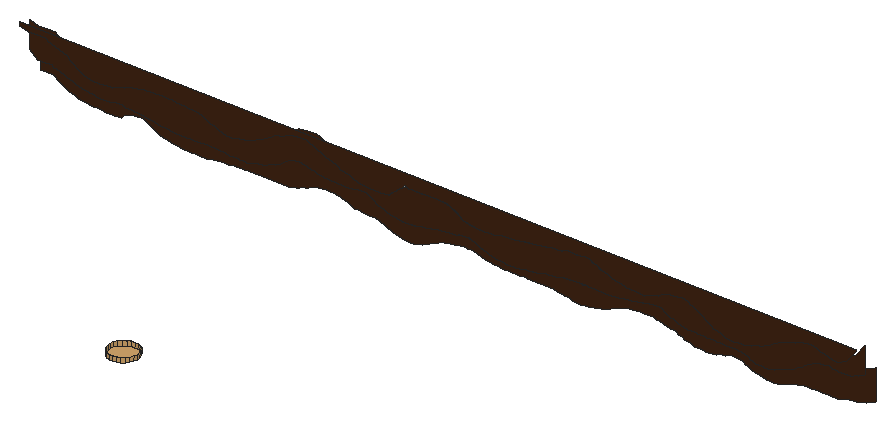
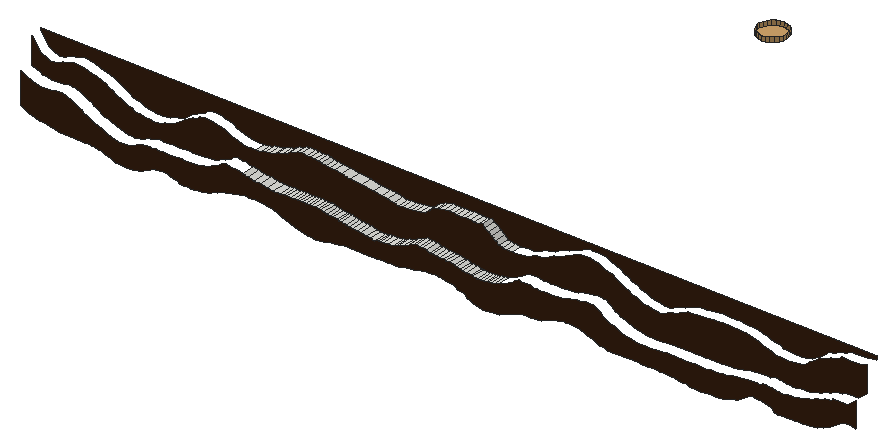
# SketchUp Ruby script. Lengths in inches.
U = 1.inch
M = Sketchup.active_model
def pt(a) = Geom::Point3d.new(a.map { |v| v * U })
def face(e, loops, mat)
  f = e.add_face(loops[0].map { |a| pt(a) })
  loops[1..].each { |l| e.add_face(l.map { |a| pt(a) }).erase! }
  f.material = f.back_material = mat if mat
  f
end
# faces: each face lists its corners as indices into pts; further lists are holes
def faces(e, pts, list, mat = nil) = list.each { |f| face(e, (f[0].is_a?(Array) ? f : [f]).map { |l| l.map { |i| pts[i] } }, mat) }
# xy, xz, yz: faces in a plane at the given z, y or x. An outline is a flat list of corners, or four numbers for a rectangle; further outlines are holes
def ring(l) = l.size == 4 ? [[l[0], l[1]], [l[2], l[1]], [l[2], l[3]], [l[0], l[3]]] : l.each_slice(2).to_a
def flat(e, list, mat, &to3) = list.each { |f| face(e, (f[0].is_a?(Array) ? f : [f]).map { |l| ring(l).map { |u, v| to3.(u, v) } }, mat) }
def xy(e, z, list, mat = nil) = flat(e, list, mat) { |x, y| [x, y, z] }
def xz(e, y, list, mat = nil) = flat(e, list, mat) { |x, z| [x, y, z] }
def yz(e, x, list, mat = nil) = flat(e, list, mat) { |y, z| [x, y, z] }
def lines(e, pts, list) = list.each { |a, b| e.add_line(pt(pts[a]), pt(pts[b])) }
# prism: a flat outline (further loops are holes) pulled along v
def prism(e, loops, v, mat = nil)
  f = face(e, loops, mat); d = Geom::Vector3d.new(v.map { |x| x * U })
  f.pushpull(f.normal.samedirection?(d) ? d.length : -d.length)
end
def box(e, o, s, mat = nil) = prism(e, [[o, [o[0] + s[0], o[1], o[2]], [o[0] + s[0], o[1] + s[1], o[2]], [o[0], o[1] + s[1], o[2]]]], [0, 0, s[2]], mat)
def at(x, y, z, deg = 0) = Geom::Transformation.translation(pt([x, y, z])) * Geom::Transformation.rotation(ORIGIN, Z_AXIS, deg.degrees)
def axes(o, x, y, z) = Geom::Transformation.new([*x, 0, *y, 0, *z, 0, *pt(o).to_a, 1])
def part(name) = M.definitions.add(name)
# library, detail: a bought-in or finely detailed component or shape, given as its bounding box
def library(name, o, s) = part(name).tap { |d| box(d.entities, o, s) }
def detail(e, o, s) = box(e.add_group.entities, o, s)
def put(e, d, t, mat = nil) = e.add_instance(d, t).tap { |i| i.material = mat if mat }
def group(e, t, mat = nil) = e.add_group.tap { |g| g.transformation = t; g.material = mat if mat }.entities
root = M.entities
M.materials.add("[Field Square Tile]").color = [211, 167, 108]
M.materials.add("[Wood Veneer 01]").color = [66, 38, 20]
xy(root,243.05,[[2994.54,563.18,2995.22,565.74]])
xy(root,243.07,[[2992.6875,563.18,2993.27,565.74]])
xy(root,243.09,[[2989.375,563.18,2989.9,565.74],[2989.9,563.18,2990.42,565.74],[2990.42,563.18,2991.08,565.74],[2991.08,563.18,2991.53,565.74]])
xy(root,249.21,[[2962.17,561.05,2963.06,563.18]])
xy(root,249.22,[[2963.78,561.05,2964.6875,563.18]])
xy(root,249.23,[[2965.33,561.05,2966.23,563.18]])
xy(root,250.6875,[[2960.72,492.77,2960.06,492.86,2959.44,493.11,2958.91,493.52,2958.5,494.05,2958.25,494.67,2958.16,495.33,2958.25,495.99,2958.5,496.61,2958.91,497.14,2959.44,497.55,2960.06,497.81,2960.72,497.89,2961.38,497.81,2962,497.55,2962.53,497.14,2962.94,496.61,2963.2,495.99,2963.28,495.33,2963.2,494.67,2962.94,494.05,2962.53,493.52,2962,493.11,2961.38,492.86]],"[Field Square Tile]")
xz(root,561.05,[[3020.59,244.87,3021.5,245.01,3022.4375,245.12,3023.2,245.25,3023.96,245.41,3024.59,245.78,3025.39,245.88,3026.1,246.16,3026.7,246.57,3027.49,246.9,3028.09,247.35,3028.76,247.62,3029.35,248.06,3030.11,248.32,3031.22,248.66,3032,248.79,3032.86,249.19,3033.53,249.32,3034.46,249.41,3035.31,249.48,3036.06,249.21,3036.7,248.96,3037.4,248.9,3038.2,248.42,3038.91,248.3,3039.62,248.22,3040.4375,248.56,3041.37,249.02,3043.1,251.16,3043.1,251.5,2889.09,251.5,2889.09,250.88,2890.68,250.53,2892.3,250.54,2893.76,250.55,2894.29,250.15,2894.9,249.97,2895.7,249.8,2896.37,249.41,2897.04,249.2,2897.81,249.01,2898.3,248.51,2898.93,248.07,2899.58,247.72,2900.22,247.25,2900.77,246.88,2901.49,246.73,2902.15,246.62,2902.89,246.54,2903.67,246.51,2904.45,246.58,2905.25,246.59,2906.05,246.69,2906.76,247.03,2907.45,247.2,2908.42,247.39,2909.05,247.78,2909.83,247.89,2910.83,248.18,2911.47,248.29,2912.36,248.35,2913.09,248.4,2914.08,248.4375,2914.74,248.46,2915.63,248.47,2916.37,248.48,2917.26,248.49,2917.99,248.39,2919.39,248.28,2920.42,248.15,2921.24,248.11,2922.04,248.08,2922.88,247.66,2923.51,247.46,2924.19,247.08,2924.875,246.94,2925.73,246.66,2926.34,246.35,2927.11,246.05,2928.01,246.13,2928.72,246.29,2929.52,246.41,2930.43,246.55,2931.16,246.92,2931.77,247.12,2932.45,247.31,2933.02,247.71,2933.95,248.03,2934.66,248.46,2935.44,248.82,2936.16,249.37,2936.95,249.5625,2937.85,249.9,2938.77,250.35,2939.43,250.49,2940.24,250.6,2941.26,250.58,2941.9,250.61,2942.52,250.32,2943.21,250.0625,2943.87,249.68,2944.63,249.46,2945.52,248.95,2946.74,248.69,2947.65,248.26,2948.25,247.9,2949.38,247.66,2949.96,247.53,2950.64,247.25,2951.45,246.95,2952.14,246.75,2952.93,246.66,2953.64,246.59,2954.53,246.55,2955.46,246.63,2956.2,246.74,2956.93,246.87,2957.54,247.42,2958.21,247.96,2958.78,248.44,2959.52,248.85,2959.99,249.34,2960.72,249.125,2961.49,249.17,2962.17,249.21,2963.06,249.21,2963.78,249.22,2964.6875,249.22,2965.33,249.23,2966.23,249.23,2966.97,249.24,2967.77,249.14,2968.4,248.82,2969.19,248.54,2969.89,248.04,2970.58,247.48,2971.47,247.29,2972.29,247.15,2973.02,247.05,2973.74,247,2974.65,246.96,2975.375,246.94,2976.29,247.04,2977.35,247.36,2978.53,247.43,2980.18,247.6,2982.16,247.98,2984.36,248.1875,2985.97,248.49,2987.22,248.62,2988.16,248.69,2988.84,248.75,2989.5,249.09,2990.2,249.18,2990.98,249.13,2991.68,249.17,2992.38,249.18,2993.28,249.29,2994.01,249.21,2994.62,248.8,2995.3125,248.73,2996.09,248.26,2996.79,248.02,2997.59,247.8125,2998.3,247.4,2999.21,247.27,2999.95,247.18,3000.875,246.91,3001.74,246.84,3002.69,246.79,3003.47,246.75,3004.22,246.83,3005.26,247.25,3006.13,247.55,3006.8,247.66,3007.43,248.16,3008.22,248.41,3008.92,248.52,3009.62,248.72,3010.32,248.8,3011.21,248.85,3012.04,248.6875,3012.58,248.26,3013.27,248.06,3014.16,247.55,3014.87,247.19,3015.68,246.63,3016.3125,246.13,3016.9,245.83,3017.58,245.67,3018.45,245.46,3019.16,245.0625,3019.875,244.95]],"[Wood Veneer 01]")
xz(root,563.18,[[3024.59,241.09,3025.16,241.14,3025.8,241.35,3026.39,241.46,3027.33,241.85,3028.33,242.23,3028.89,242.42,3029.61,242.61,3030.125,242.91,3030.5,243.14,3031.04,243.52,3031.52,243.71,3031.85,244.02,3032.29,244.21,3032.88,244.57,3033.35,244.76,3033.97,245.125,3034.47,245.32,3034.95,245.41,3035.5,245.48,3035.99,245.59,3036.52,245.55,3037.13,245.35,3037.62,245.31,3038.17,245.27,3038.73,245.24,3039.29,245.22,3039.85,245.34,3040.48,245.42,3041.0625,245.52,3041.44,245.76,3041.91,245.9,3043.1,246.43,3043.1,251.16,3041.37,249.02,3040.4375,248.56,3039.62,248.22,3038.91,248.3,3038.2,248.42,3037.4,248.9,3036.7,248.96,3036.06,249.21,3035.31,249.48,3034.46,249.41,3033.53,249.32,3032.86,249.19,3032,248.79,3031.22,248.66,3030.11,248.32,3029.35,248.06,3028.76,247.62,3028.09,247.35,3027.49,246.9,3026.7,246.57,3026.1,246.16,3025.39,245.88,3024.59,245.78,3023.96,245.41,3023.2,245.25,3022.4375,245.12,3021.5,245.01,3020.59,244.87,3019.875,244.95,3019.16,245.0625,3018.45,245.46,3017.58,245.67,3016.9,245.83,3016.3125,246.13,3015.68,246.63,3014.87,247.19,3014.16,247.55,3013.27,248.06,3012.58,248.26,3012.04,248.6875,3011.21,248.85,3010.32,248.8,3009.62,248.72,3008.92,248.52,3008.22,248.41,3007.43,248.16,3006.8,247.66,3006.13,247.55,3005.26,247.25,3004.22,246.83,3003.47,246.75,3002.69,246.79,3001.74,246.84,3000.875,246.91,2999.95,247.18,2999.21,247.27,2998.3,247.4,2997.59,247.8125,2996.79,248.02,2996.09,248.26,2995.3125,248.73,2994.62,248.8,2994.01,249.21,2993.28,249.29,2992.38,249.18,2991.68,249.17,2990.98,249.13,2990.2,249.18,2989.5,249.09,2988.84,248.75,2988.16,248.69,2987.22,248.62,2985.97,248.49,2984.36,248.1875,2982.16,247.98,2980.18,247.6,2978.53,247.43,2977.35,247.36,2976.29,247.04,2975.375,246.94,2974.65,246.96,2973.74,247,2973.02,247.05,2972.29,247.15,2971.47,247.29,2970.58,247.48,2969.89,248.04,2969.19,248.54,2968.4,248.82,2967.77,249.14,2966.97,249.24,2966.23,249.23,2965.33,249.23,2964.6875,249.22,2963.78,249.22,2963.06,249.21,2962.17,249.21,2961.49,249.17,2960.72,249.125,2959.99,249.34,2959.52,248.85,2958.78,248.44,2958.21,247.96,2957.54,247.42,2956.93,246.87,2956.2,246.74,2955.46,246.63,2954.53,246.55,2953.64,246.59,2952.93,246.66,2952.14,246.75,2951.45,246.95,2950.64,247.25,2949.96,247.53,2949.38,247.66,2948.25,247.9,2947.65,248.26,2946.74,248.69,2945.52,248.95,2944.63,249.46,2943.87,249.68,2943.21,250.0625,2942.52,250.32,2941.9,250.61,2941.26,250.58,2940.24,250.6,2939.43,250.49,2938.77,250.35,2937.85,249.9,2936.95,249.5625,2936.16,249.37,2935.44,248.82,2934.66,248.46,2933.95,248.03,2933.02,247.71,2932.45,247.31,2931.77,247.12,2931.16,246.92,2930.43,246.55,2929.52,246.41,2928.72,246.29,2928.01,246.13,2927.11,246.05,2926.34,246.35,2925.73,246.66,2924.875,246.94,2924.19,247.08,2923.51,247.46,2922.88,247.66,2922.04,248.08,2921.24,248.11,2920.42,248.15,2919.39,248.28,2917.99,248.39,2917.26,248.49,2916.37,248.48,2915.63,248.47,2914.74,248.46,2914.08,248.4375,2913.09,248.4,2912.36,248.35,2911.47,248.29,2910.83,248.18,2909.83,247.89,2909.05,247.78,2908.42,247.39,2907.45,247.2,2906.76,247.03,2906.05,246.69,2905.25,246.59,2904.45,246.58,2903.67,246.51,2902.89,246.54,2902.15,246.62,2901.49,246.73,2900.77,246.88,2900.22,247.25,2899.58,247.72,2898.93,248.07,2898.3,248.51,2897.81,249.01,2897.04,249.2,2896.37,249.41,2895.7,249.8,2894.9,249.97,2894.29,250.15,2893.76,250.55,2892.3,250.54,2890.68,250.53,2889.09,250.88,2889.09,246.2,2890.66,244.96,2892.05,244.9375,2893.3,244.92,2893.52,244.61,2894.08,244.54,2894.84,244.41,2895.51,244.11,2896.03,243.95,2896.69,243.79,2897.21,243.48,2897.85,243.3,2898.4375,243.14,2898.92,243.06,2899.64,242.85,2900.22,242.78,2901.03,242.73,2901.57,242.68,2902.24,242.51,2902.76,242.46,2903.3,242.58,2903.93,242.57,2904.56,242.81,2905.13,242.86,2905.69,242.89,2906.33,242.92,2906.76,242.625,2907.37,242.65,2907.92,242.62,2908.55,242.58,2909.11,242.57,2909.75,242.48,2910.41,242.38,2911.07,242.34,2911.74,242.24,2912.91,241.96,2913.68,241.89,2914.5,241.83,2915.1,241.78,2915.87,241.75,2916.32,241.74,2916.87,241.72,2918.13,241.7,2918.86,241.69,2919.53,241.68,2920.12,241.68,2920.61,241.67,2921.3125,241.74,2921.88,241.75,2923.88,241.75,2924.37,241.67,2924.9,241.66,2925.51,241.57,2926.05,241.53,2926.67,241.51,2927.22,241.49,2927.92,241.48,2928.58,241.47,2929.15,241.46,2929.86,241.6,2930.59,241.85,2931.26,241.91,2932.16,242.1,2932.93,242.46,2933.63,242.78,2934.4,242.97,2934.93,243.23,2935.33,243.48,2935.85,243.72,2936.1875,244.12,2936.66,244.39,2937.14,244.73,2937.625,244.87,2938.21,244.95,2938.89,245.01,2939.54,244.81,2940.11,244.7,2940.59,244.67,2941.2,244.55,2941.74,244.51,2942.2,244.25,2942.95,244.11,2943.51,244.04,2944.13,243.99,2944.85,243.95,2945.35,243.93,2946.04,243.91,2946.61,243.89,2947.31,243.88,2947.96,243.94,2948.6,243.95,2949.16,244.1,2949.79,244.13,2950.27,244.15,2950.79,244.17,2951.31,244.18,2951.91,243.8,2952.45,243.43,2953.06,243.09,2953.45,242.875,2953.95,242.68,2954.54,242.51,2955.05,242.21,2955.65,242.11,2956.33,241.96,2956.89,241.89,2957.35,241.85,2957.87,241.8125,2958.38,241.79,2958.96,241.78,2959.63,241.91,2960.1,241.93,2960.77,242.09,2961.54,242.2,2962.04,242.24,2962.65,242.42,2963.2,242.47,2963.95,242.71,2964.59,242.78,2965.07,242.82,2965.76,242.85,2966.46,242.87,2967.01,243.02,2967.63,243.05,2968.18,243.29,2968.86,243.35,2969.41,243.39,2970.01,243.42,2970.78,243.14,2971.35,242.9375,2971.9,242.65,2972.52,242.39,2973.28,242.14,2973.92,241.89,2974.41,241.78,2975.46,241.63,2976.23,241.56,2976.83,241.51,2977.28,241.48,2977.8,241.46,2978.67,241.51,2979.39,241.59,2980.33,241.82,2981.11,241.87,2981.875,241.98,2982.49,242.02,2983.14,242.19,2983.84,242.38,2984.33,242.4375,2984.85,242.48,2985.51,242.58,2986.04,242.61,2986.625,242.77,2987.08,242.95,2987.64,243.01,2988.15,243.05,2988.72,243.08,2989.375,243.09,2991.53,243.09,2992.1,243.08,2992.6875,243.07,2993.27,243.07,2993.93,243.0625,2994.54,243.05,2995.22,243.05,2996.49,243.1,2997.66,243.17,2998.8,243.4,3000.0625,243.52,3001.19,243.71,3002.09,243.99,3002.79,244.08,3003.49,244.21,3004.07,244.27,3004.61,244.3,3005.28,244.39,3005.875,244.19,3006.25,243.88,3006.73,243.59,3007.28,243.33,3007.83,243.22,3008.32,242.92,3008.8,242.75,3009.36,242.6,3009.92,242.52,3010.48,242.47,3011.0625,242.43,3011.64,242.4,3012.22,242.39,3012.8,242.37,3013.38,242.36,3013.97,242.35,3015.13,242.33,3015.71,242.33,3016.43,242.32,3016.9,242.3125,3017.54,242.3,3018.21,242.3,3018.66,242.29,3019.3,242.28,3019.8125,242.28,3020.44,242.2,3021.02,241.97,3021.59,241.84,3022.1,241.57,3022.52,241.33,3022.99,241.24,3023.52,241.17,3023.99,241.12]],"[Wood Veneer 01]")
xz(root,565.74,[[2957.95,236.98,2958.63,237.22,2959.48,237.43,2960.1,237.74,2960.8,238.02,2961.24,238.375,2961.8,238.51,2962.4375,238.76,2963.08,239.12,2963.66,239.22,2964.66,239.31,2965.47,239.54,2965.96,239.6,2966.58,239.65,2967.17,239.69,2967.73,239.7,2968.46,239.72,2969.07,239.56,2969.74,239.44,2970.59,239.16,2971.14,239.07,2971.91,238.93,2972.79,238.78,2973.27,238.73,2973.94,238.6875,2974.63,238.66,2975.3,238.65,2976.08,238.64,2976.7,238.63,2977.39,238.625,2978.25,238.625,2978.81,238.62,2983.7,238.62,2984.39,238.45,2985.15,238.25,2985.77,238.19,2986.54,238.15,2987.17,237.86,2987.94,237.79,2988.65,237.74,2989.52,237.87,2990.17,237.88,2991.29,238.14,2992.51,238.46,2993.26,238.72,2994.14,239.08,2994.93,239.375,2995.67,239.75,2996.32,239.97,2996.94,240.17,2997.62,240.27,2998.3,240.33,2998.99,240.37,2999.68,240.4,3000.375,240.41,3000.9,240.42,3001.48,240.43,3002.05,240.43,3002.7,240.27,3003.28,240.23,3003.93,239.96,3004.6875,239.8,3005.3,239.65,3006.0625,239.5,3006.6875,239.18,3007.37,239.01,3007.89,238.67,3008.46,238.56,3009.12,238.48,3009.6875,238.26,3010.26,238.19,3011.08,238.15,3011.61,238.11,3012.28,238.18,3012.96,238.18,3013.64,238.27,3014.16,238.55,3014.82,238.61,3015.41,238.66,3015.98,239.04,3016.72,239.125,3017.4,239.02,3018.09,238.96,3018.61,238.86,3019.11,238.57,3019.66,238.33,3020.37,238,3021.2,237.71,3021.74,237.59,3022.34,237.51,3022.93,237.45,3023.5,237.42,3024.23,237.4,3024.91,237.47,3025.51,237.5625,3026.2,237.84,3026.88,238.08,3027.57,238.33,3028.1,238.51,3028.67,238.6,3029.33,238.74,3029.91,238.8,3030.48,238.83,3031.22,238.86,3031.98,238.875,3032.52,238.88,3033.2,238.89,3033.88,238.89,3034.64,238.9,3036.03,238.9,3036.66,239.15,3037.43,239.28,3038.23,239.42,3038.95,239.49,3039.5,239.53,3040.1875,239.81,3040.71,239.96,3041.27,240.1,3043.1,240.89,3043.1,246.43,3041.91,245.9,3041.44,245.76,3041.0625,245.52,3040.48,245.42,3039.85,245.34,3039.29,245.22,3038.73,245.24,3038.17,245.27,3037.62,245.31,3037.13,245.35,3036.52,245.55,3035.99,245.59,3035.5,245.48,3034.95,245.41,3034.47,245.32,3033.97,245.125,3033.35,244.76,3032.88,244.57,3032.29,244.21,3031.85,244.02,3031.52,243.71,3031.04,243.52,3030.5,243.14,3030.125,242.91,3029.61,242.61,3028.89,242.42,3028.33,242.23,3027.33,241.85,3026.39,241.46,3025.8,241.35,3025.16,241.14,3024.59,241.09,3023.99,241.12,3023.52,241.17,3022.99,241.24,3022.52,241.33,3022.1,241.57,3021.59,241.84,3021.02,241.97,3020.44,242.2,3019.8125,242.28,3019.3,242.28,3018.66,242.29,3018.21,242.3,3017.54,242.3,3016.9,242.3125,3016.43,242.32,3015.71,242.33,3015.13,242.33,3013.97,242.35,3013.38,242.36,3012.8,242.37,3012.22,242.39,3011.64,242.4,3011.0625,242.43,3010.48,242.47,3009.92,242.52,3009.36,242.6,3008.8,242.75,3008.32,242.92,3007.83,243.22,3007.28,243.33,3006.73,243.59,3006.25,243.88,3005.875,244.19,3005.28,244.39,3004.61,244.3,3004.07,244.27,3003.49,244.21,3002.79,244.08,3002.09,243.99,3001.19,243.71,3000.0625,243.52,2998.8,243.4,2997.66,243.17,2996.49,243.1,2995.22,243.05,2994.54,243.05,2993.93,243.0625,2993.27,243.07,2992.6875,243.07,2992.1,243.08,2991.53,243.09,2989.375,243.09,2988.72,243.08,2988.15,243.05,2987.64,243.01,2987.08,242.95,2986.625,242.77,2986.04,242.61,2985.51,242.58,2984.85,242.48,2984.33,242.4375,2983.84,242.38,2983.14,242.19,2982.49,242.02,2981.875,241.98,2981.11,241.87,2980.33,241.82,2979.39,241.59,2978.67,241.51,2977.8,241.46,2977.28,241.48,2976.83,241.51,2976.23,241.56,2975.46,241.63,2974.41,241.78,2973.92,241.89,2973.28,242.14,2972.52,242.39,2971.9,242.65,2971.35,242.9375,2970.78,243.14,2970.01,243.42,2969.41,243.39,2968.86,243.35,2968.18,243.29,2967.63,243.05,2967.01,243.02,2966.46,242.87,2965.76,242.85,2965.07,242.82,2964.59,242.78,2963.95,242.71,2963.2,242.47,2962.65,242.42,2962.04,242.24,2961.54,242.2,2960.77,242.09,2960.1,241.93,2959.63,241.91,2958.96,241.78,2958.38,241.79,2957.87,241.8125,2957.35,241.85,2956.89,241.89,2956.33,241.96,2955.65,242.11,2955.05,242.21,2954.54,242.51,2953.95,242.68,2953.45,242.875,2953.06,243.09,2952.45,243.43,2951.91,243.8,2951.31,244.18,2950.79,244.17,2950.27,244.15,2949.79,244.13,2949.16,244.1,2948.6,243.95,2947.96,243.94,2947.31,243.88,2946.61,243.89,2946.04,243.91,2945.35,243.93,2944.85,243.95,2944.13,243.99,2943.51,244.04,2942.95,244.11,2942.2,244.25,2941.74,244.51,2941.2,244.55,2940.59,244.67,2940.11,244.7,2939.54,244.81,2938.89,245.01,2938.21,244.95,2937.625,244.87,2937.14,244.73,2936.66,244.39,2936.1875,244.12,2935.85,243.72,2935.33,243.48,2934.93,243.23,2934.4,242.97,2933.63,242.78,2932.93,242.46,2932.16,242.1,2931.26,241.91,2930.59,241.85,2929.86,241.6,2929.15,241.46,2928.58,241.47,2927.92,241.48,2927.22,241.49,2926.67,241.51,2926.05,241.53,2925.51,241.57,2924.9,241.66,2924.37,241.67,2923.88,241.75,2921.88,241.75,2921.3125,241.74,2920.61,241.67,2920.12,241.68,2919.53,241.68,2918.86,241.69,2918.13,241.7,2916.87,241.72,2916.32,241.74,2915.87,241.75,2915.1,241.78,2914.5,241.83,2913.68,241.89,2912.91,241.96,2911.74,242.24,2911.07,242.34,2910.41,242.38,2909.75,242.48,2909.11,242.57,2908.55,242.58,2907.92,242.62,2907.37,242.65,2906.76,242.625,2906.33,242.92,2905.69,242.89,2905.13,242.86,2904.56,242.81,2903.93,242.57,2903.3,242.58,2902.76,242.46,2902.24,242.51,2901.57,242.68,2901.03,242.73,2900.22,242.78,2899.64,242.85,2898.92,243.06,2898.4375,243.14,2897.85,243.3,2897.21,243.48,2896.69,243.79,2896.03,243.95,2895.51,244.11,2894.84,244.41,2894.08,244.54,2893.52,244.61,2893.3,244.92,2892.05,244.9375,2890.66,244.96,2889.09,246.2,2889.09,241.52,2890.3,241.69,2891.57,241.55,2892.59,240.85,2893.13,240.59,2893.73,240.2,2894.52,239.86,2894.97,239.64,2895.53,239.52,2896.04,239.19,2896.82,239.09,2897.51,239.03,2898.19,238.97,2898.89,238.94,2899.59,238.93,2900.28,238.92,2901.32,238.82,2901.83,238.8,2902.7,238.79,2903.44,238.77,2903.97,238.9375,2904.53,239.55,2905.11,239.69,2905.66,239.88,2906.39,239.99,2906.98,240.05,2907.64,240.09,2908.33,240.11,2909.03,239.71,2909.49,239.38,2910.07,239.11,2910.65,238.74,2911.3,238.43,2912.21,238.31,2912.68,238.21,2913.62,237.9,2914.28,237.82,2914.97,237.76,2915.68,237.71,2916.29,237.68,2916.89,237.67,2917.64,237.66,2918.33,237.65,2919.64,237.65,2920.31,237.89,2921.07,237.94,2921.6875,237.98,2922.54,238.1,2923.09,238.13,2923.85,238.15,2924.48,238.26,2925.23,238.28,2925.86,238.3,2926.71,238.32,2927.43,238.33,2928.66,238.33,2929.34,238.34,2934.91,238.34,2935.42,238.59,2936.24,238.72,2936.93,238.86,2937.44,239.18,2938.03,239.35,2938.59,239.52,2939.14,239.85,2939.78,240.03,2940.4375,240.12,2941.11,240.19,2941.875,240.23,2942.58,240.25,2943.2,240.27,2943.98,240.11,2944.61,239.92,2945.3,239.7,2945.83,239.53,2946.41,239.29,2947.07,239.04,2947.65,238.94,2948.22,238.875,2948.97,238.83,2949.73,238.8,2950.27,238.79,2950.94,238.78,2951.72,238.43,2952.5,238.28,2953.0625,237.96,2954,237.68,2954.67,237.33,2955.2,237.2,2955.89,237.11,2956.65,237.04,2957.34,237.01]],"[Wood Veneer 01]")
p = [[2976.23,563.18,241.56],[2976.23,565.74,241.56],[2976.83,565.74,241.51],[2976.83,563.18,241.51],[2977.28,565.74,241.48],[2977.28,563.18,241.48],
  [2977.8,565.74,241.46],[2977.8,563.18,241.46],[2978.67,565.74,241.51],[2978.67,563.18,241.51],[2979.39,565.74,241.59],[2979.39,563.18,241.59],
  [2974.41,563.18,241.78],[2974.41,565.74,241.78],[2975.46,565.74,241.63],[2975.46,563.18,241.63],[2980.33,565.74,241.82],[2980.33,563.18,241.82],
  [2956.89,563.18,241.89],[2956.89,565.74,241.89],[2957.35,565.74,241.85],[2957.35,563.18,241.85],[2957.87,565.74,241.8125],[2957.87,563.18,241.8125],
  [2958.38,565.74,241.79],[2958.38,563.18,241.79],[2958.96,565.74,241.78],[2958.96,563.18,241.78],[2959.63,565.74,241.91],[2959.63,563.18,241.91],
  [2973.92,563.18,241.89],[2973.92,565.74,241.89],[2981.11,565.74,241.87],[2981.11,563.18,241.87],[2956.33,563.18,241.96],[2956.33,565.74,241.96],
  [2960.1,565.74,241.93],[2960.1,563.18,241.93],[2960.77,565.74,242.09],[2960.77,563.18,242.09],[2973.28,563.18,242.14],[2973.28,565.74,242.14],
  [2981.875,565.74,241.98],[2981.875,563.18,241.98],[2955.65,563.18,242.11],[2955.65,565.74,242.11],[2982.49,565.74,242.02],[2982.49,563.18,242.02],
  [2983.14,565.74,242.19],[2983.14,563.18,242.19],[2955.05,563.18,242.21],[2955.05,565.74,242.21],[2961.54,565.74,242.2],[2961.54,563.18,242.2],
  [2972.52,563.18,242.39],[2972.52,565.74,242.39],[2962.04,565.74,242.24],[2962.04,563.18,242.24],[2962.65,565.74,242.42],[2962.65,563.18,242.42],
  [2983.84,565.74,242.38],[2983.84,563.18,242.38],[2963.2,565.74,242.47],[2963.2,563.18,242.47],[2971.9,563.18,242.65],[2971.9,565.74,242.65],
  [2984.33,565.74,242.4375],[2984.33,563.18,242.4375],[2984.85,565.74,242.48],[2984.85,563.18,242.48],[2963.95,565.74,242.71],[2963.95,563.18,242.71],
  [2985.51,565.74,242.58],[2985.51,563.18,242.58],[2971.35,563.18,242.9375],[2971.35,565.74,242.9375],[2986.04,565.74,242.61],[2986.04,563.18,242.61],
  [2986.625,565.74,242.77],[2986.625,563.18,242.77],[2964.59,565.74,242.78],[2964.59,563.18,242.78],[2965.07,565.74,242.82],[2965.07,563.18,242.82],
  [2965.76,565.74,242.85],[2965.76,563.18,242.85],[2987.08,565.74,242.95],[2987.08,563.18,242.95],[2966.46,565.74,242.87],[2966.46,563.18,242.87],
  [2967.01,565.74,243.02],[2967.01,563.18,243.02],[2970.78,563.18,243.14],[2970.78,565.74,243.14],[2967.63,565.74,243.05],[2967.63,563.18,243.05],
  [2987.64,565.74,243.01],[2987.64,563.18,243.01],[2988.15,565.74,243.05],[2988.15,563.18,243.05],[2988.72,565.74,243.08],[2988.72,563.18,243.08],
  [2995.22,563.18,243.05],[2995.22,565.74,243.05],[2996.49,565.74,243.1],[2996.49,563.18,243.1],[2968.18,565.74,243.29],[2968.18,563.18,243.29],
  [2970.01,563.18,243.42],[2970.01,565.74,243.42],[2989.375,565.74,243.09],[2989.375,563.18,243.09],[2991.53,563.18,243.09],[2991.53,565.74,243.09],
  [2992.1,565.74,243.08],[2992.1,563.18,243.08],[2992.6875,565.74,243.07],[2992.6875,563.18,243.07],[2993.27,563.18,243.07],[2993.27,565.74,243.07],
  [2993.93,565.74,243.0625],[2993.93,563.18,243.0625],[2994.54,565.74,243.05],[2994.54,563.18,243.05],[2997.66,565.74,243.17],[2997.66,563.18,243.17],
  [2998.8,565.74,243.4],[2998.8,563.18,243.4],[2968.86,565.74,243.35],[2968.86,563.18,243.35],[2969.41,565.74,243.39],[2969.41,563.18,243.39],
  [3000.0625,565.74,243.52],[3000.0625,563.18,243.52],[3001.19,565.74,243.71],[3001.19,563.18,243.71],[3002.09,565.74,243.99],[3002.09,563.18,243.99],
  [2954.53,561.05,246.55],[2954.53,563.18,246.55],[2955.46,563.18,246.63],[2955.46,561.05,246.63],[2956.2,563.18,246.74],[2956.2,561.05,246.74],
  [2956.93,563.18,246.87],[2956.93,561.05,246.87],[3000.875,561.05,246.91],[3000.875,563.18,246.91],[3001.74,563.18,246.84],[3001.74,561.05,246.84],
  [2957.54,563.18,247.42],[2957.54,561.05,247.42],[2974.65,561.05,246.96],[2974.65,563.18,246.96],[2975.375,563.18,246.94],[2975.375,561.05,246.94],
  [2976.29,563.18,247.04],[2976.29,561.05,247.04],[2999.95,561.05,247.18],[2999.95,563.18,247.18],[2972.29,561.05,247.15],[2972.29,563.18,247.15],
  [2973.02,563.18,247.05],[2973.02,561.05,247.05],[2973.74,563.18,247],[2973.74,561.05,247],[2977.35,563.18,247.36],[2977.35,561.05,247.36],
  [2971.47,561.05,247.29],[2971.47,563.18,247.29],[2999.21,561.05,247.27],[2999.21,563.18,247.27],[2970.58,561.05,247.48],[2970.58,563.18,247.48],
  [2998.3,561.05,247.4],[2998.3,563.18,247.4],[2958.21,563.18,247.96],[2958.21,561.05,247.96],[2978.53,563.18,247.43],[2978.53,561.05,247.43],
  [2980.18,563.18,247.6],[2980.18,561.05,247.6],[2997.59,561.05,247.8125],[2997.59,563.18,247.8125],[2969.89,561.05,248.04],[2969.89,563.18,248.04],
  [2982.16,563.18,247.98],[2982.16,561.05,247.98],[2996.79,561.05,248.02],[2996.79,563.18,248.02],[2958.78,563.18,248.44],[2958.78,561.05,248.44],
  [2969.19,561.05,248.54],[2969.19,563.18,248.54],[2984.36,563.18,248.1875],[2984.36,561.05,248.1875],[2996.09,561.05,248.26],[2996.09,563.18,248.26],
  [2985.97,563.18,248.49],[2985.97,561.05,248.49],[2995.3125,561.05,248.73],[2995.3125,563.18,248.73],[2959.52,563.18,248.85],[2959.52,561.05,248.85],
  [2968.4,561.05,248.82],[2968.4,563.18,248.82],[2987.22,563.18,248.62],[2987.22,561.05,248.62],[2988.16,563.18,248.69],[2988.16,561.05,248.69],
  [2988.84,563.18,248.75],[2988.84,561.05,248.75],[2994.62,561.05,248.8],[2994.62,563.18,248.8],[2967.77,561.05,249.14],[2967.77,563.18,249.14],
  [2989.5,563.18,249.09],[2989.5,561.05,249.09],[2994.01,561.05,249.21],[2994.01,563.18,249.21],[2959.99,563.18,249.34],[2959.99,561.05,249.34],
  [2960.72,563.18,249.125],[2960.72,561.05,249.125],[2961.49,563.18,249.17],[2961.49,561.05,249.17],[2966.97,561.05,249.24],[2966.97,563.18,249.24],
  [2990.2,563.18,249.18],[2990.2,561.05,249.18],[2990.98,563.18,249.13],[2990.98,561.05,249.13],[2991.68,563.18,249.17],[2991.68,561.05,249.17],
  [2962.17,563.18,249.21],[2962.17,561.05,249.21],[2963.06,561.05,249.21],[2963.06,563.18,249.21],[2963.78,563.18,249.22],[2963.78,561.05,249.22],
  [2964.6875,561.05,249.22],[2964.6875,563.18,249.22],[2965.33,563.18,249.23],[2965.33,561.05,249.23],[2966.23,561.05,249.23],[2966.23,563.18,249.23],
  [2992.38,563.18,249.18],[2992.38,561.05,249.18],[2993.28,563.18,249.29],[2993.28,561.05,249.29],[2960.72,492.77,251.5],[2960.06,492.86,251.5],
  [2960.06,492.86,250.6875],[2960.72,492.77,250.6875],[2961.38,492.86,251.5],[2961.38,492.86,250.6875],[2959.44,493.11,251.5],[2959.44,493.11,250.6875],
  [2962,493.11,251.5],[2962,493.11,250.6875],[2958.91,493.52,251.5],[2958.91,493.52,250.6875],[2962.53,493.52,251.5],[2962.53,493.52,250.6875],
  [2958.5,494.05,251.5],[2958.5,494.05,250.6875],[2962.94,494.05,251.5],[2962.94,494.05,250.6875],[2958.25,494.67,251.5],[2958.25,494.67,250.6875],
  [2963.2,494.67,251.5],[2963.2,494.67,250.6875],[2958.16,495.33,251.5],[2958.16,495.33,250.6875],[2963.28,495.33,251.5],[2963.28,495.33,250.6875],
  [2958.25,495.99,251.5],[2958.25,495.99,250.6875],[2963.2,495.99,251.5],[2963.2,495.99,250.6875],[2958.5,496.61,251.5],[2958.5,496.61,250.6875],
  [2962.94,496.61,251.5],[2962.94,496.61,250.6875],[2958.91,497.14,251.5],[2958.91,497.14,250.6875],[2962.53,497.14,251.5],[2962.53,497.14,250.6875],
  [2959.44,497.55,251.5],[2959.44,497.55,250.6875],[2962,497.55,251.5],[2962,497.55,250.6875],[2960.06,497.81,251.5],[2960.06,497.81,250.6875],
  [2961.38,497.81,251.5],[2961.38,497.81,250.6875],[2960.72,497.89,251.5],[2960.72,497.89,250.6875]]
faces(root,p,[[0,1,2,3],[3,2,4,5],[5,4,6,7],[7,6,8,9],[9,8,10,11],[12,13,14,15],[15,14,1,0],[11,10,16,17],
  [18,19,20,21],[21,20,22,23],[23,22,24,25],[25,24,26,27],[27,26,28,29],[30,31,13,12],[17,16,32,33],[34,35,19,18],
  [29,28,36,37],[37,36,38,39],[40,41,31,30],[33,32,42,43],[44,45,35,34],[43,42,46,47],[47,46,48,49],[50,51,45,44],
  [39,38,52,53],[54,55,41,40],[53,52,56,57],[57,56,58,59],[49,48,60,61],[59,58,62,63],[64,65,55,54],[61,60,66,67],
  [67,66,68,69],[63,62,70,71],[69,68,72,73],[74,75,65,64],[73,72,76,77],[77,76,78,79],[71,70,80,81],[81,80,82,83],
  [83,82,84,85],[79,78,86,87],[85,84,88,89],[89,88,90,91],[92,93,75,74],[91,90,94,95],[87,86,96,97],[97,96,98,99],
  [99,98,100,101],[102,103,104,105],[95,94,106,107],[108,109,93,92],[101,100,110,111],[112,113,114,115],[115,114,116,117],[118,119,120,121],
  [121,120,122,123],[105,104,124,125],[125,124,126,127],[107,106,128,129],[129,128,130,131],[131,130,109,108],[127,126,132,133],[133,132,134,135],
  [135,134,136,137],[138,139,140,141],[141,140,142,143],[143,142,144,145],[146,147,148,149],[145,144,150,151],[152,153,154,155],[155,154,156,157],
  [158,159,147,146],[160,161,162,163],[163,162,164,165],[165,164,153,152],[157,156,166,167],[168,169,161,160],[170,171,159,158],[172,173,169,168],
  [174,175,171,170],[151,150,176,177],[167,166,178,179],[179,178,180,181],[182,183,175,174],[184,185,173,172],[181,180,186,187],[188,189,183,182],
  [177,176,190,191],[192,193,185,184],[187,186,194,195],[196,197,189,188],[195,194,198,199],[200,201,197,196],[191,190,202,203],[204,205,193,192],
  [199,198,206,207],[207,206,208,209],[209,208,210,211],[212,213,201,200],[214,215,205,204],[211,210,216,217],[218,219,213,212],[203,202,220,221],
  [221,220,222,223],[223,222,224,225],[226,227,215,214],[217,216,228,229],[229,228,230,231],[231,230,232,233],[225,224,234,235],[236,237,238,239],
  [240,241,242,243],[244,245,227,226],[233,232,246,247],[247,246,248,249],[249,248,219,218]])
faces(root,p,[[250,251,252,253],[254,250,253,255],[251,256,257,252],[258,254,255,259],[256,260,261,257],[262,258,259,263],[260,264,265,261],[266,262,263,267],
  [264,268,269,265],[270,266,267,271],[268,272,273,269],[274,270,271,275],[272,276,277,273],[278,274,275,279],[276,280,281,277],[282,278,279,283],
  [280,284,285,281],[286,282,283,287],[284,288,289,285],[290,286,287,291],[288,292,293,289],[294,290,291,295],[292,296,297,293],[296,294,295,297]],"[Field Square Tile]")
